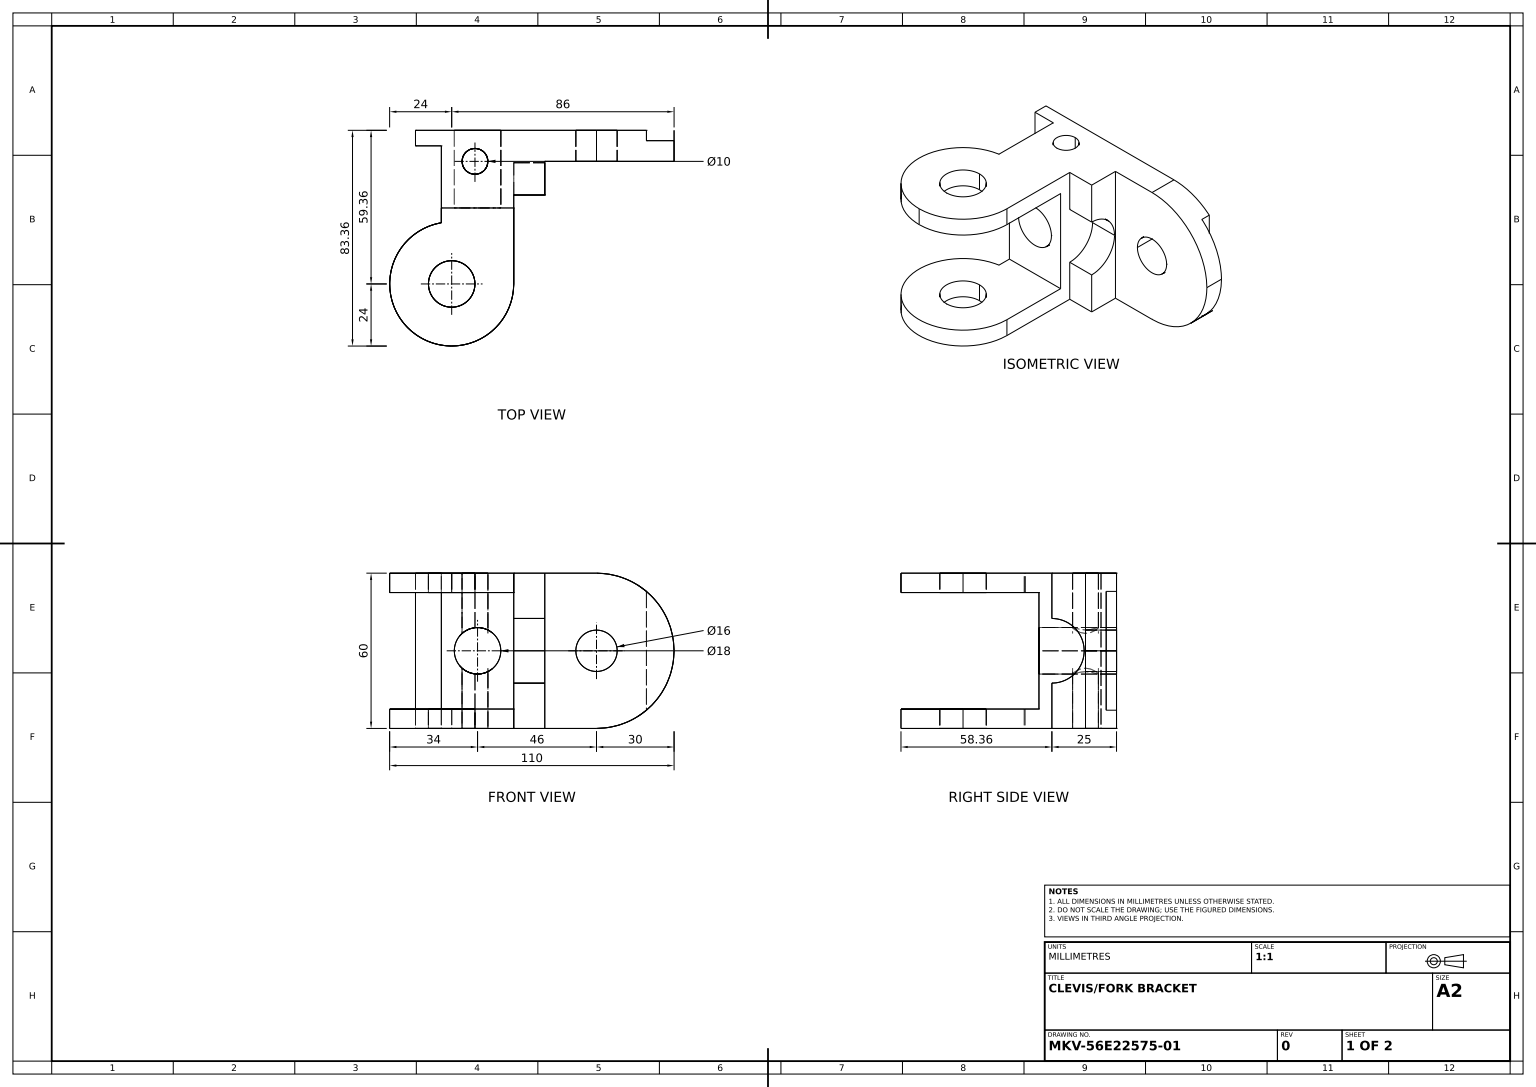
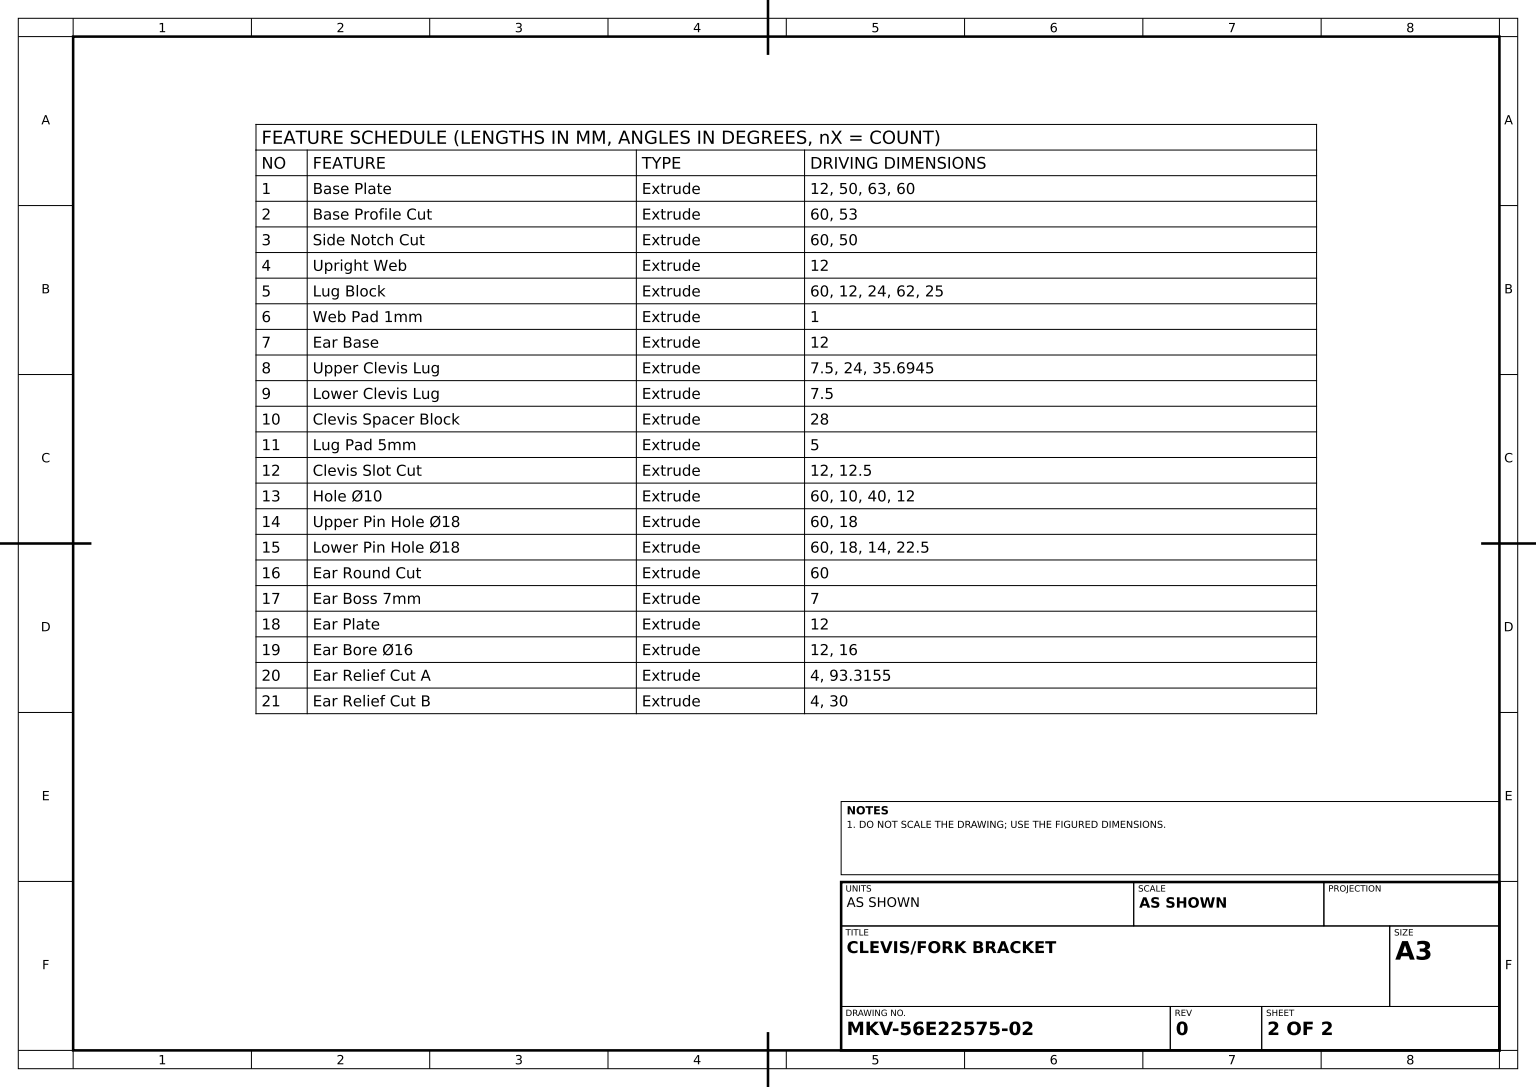
ISO-10303-21;
HEADER;
FILE_DESCRIPTION((''),'2;1');
FILE_NAME('','',(''),(''),'','','');
FILE_SCHEMA(('AUTOMOTIVE_DESIGN'));
ENDSEC;
DATA;
#1=APPLICATION_CONTEXT('');
#2=PRODUCT_CONTEXT('',#1,'mechanical');
#3=PRODUCT('','','',(#2));
#4=PRODUCT_DEFINITION_FORMATION('','',#3);
#5=PRODUCT_DEFINITION_CONTEXT('',#1,'design');
#6=PRODUCT_DEFINITION('','',#4,#5);
#7=PRODUCT_DEFINITION_SHAPE('','',#6);
#8=(LENGTH_UNIT()NAMED_UNIT(*)SI_UNIT(.MILLI.,.METRE.));
#9=(NAMED_UNIT(*)PLANE_ANGLE_UNIT()SI_UNIT($,.RADIAN.));
#10=(NAMED_UNIT(*)SI_UNIT($,.STERADIAN.)SOLID_ANGLE_UNIT());
#11=UNCERTAINTY_MEASURE_WITH_UNIT(LENGTH_MEASURE(1.E-05),#8,'distance_accuracy_value','');
#12=(GEOMETRIC_REPRESENTATION_CONTEXT(3)GLOBAL_UNCERTAINTY_ASSIGNED_CONTEXT((#11))GLOBAL_UNIT_ASSIGNED_CONTEXT((#8,#9,#10))REPRESENTATION_CONTEXT('',''));
#13=CARTESIAN_POINT('',(10.,52.5,35.694478));
#14=VERTEX_POINT('',#13);
#15=CARTESIAN_POINT('',(10.,60.,35.694478));
#16=VERTEX_POINT('',#15);
#17=DIRECTION('',(0.,1.,0.));
#18=VECTOR('',#17,1000.);
#19=LINE('',#13,#18);
#20=EDGE_CURVE('',#14,#16,#19,.T.);
#21=ORIENTED_EDGE('',*,*,#20,.T.);
#22=CARTESIAN_POINT('',(10.,60.,6.));
#23=VERTEX_POINT('',#22);
#24=CARTESIAN_POINT('',(10.,60.,0.));
#25=DIRECTION('',(0.,0.,1.));
#26=VECTOR('',#25,1000.);
#27=LINE('',#24,#26);
#28=EDGE_CURVE('',#23,#16,#27,.T.);
#29=ORIENTED_EDGE('',*,*,#28,.F.);
#30=CARTESIAN_POINT('',(10.,0.,6.));
#31=VERTEX_POINT('',#30);
#32=DIRECTION('',(0.,-1.,0.));
#33=VECTOR('',#32,1000.);
#34=LINE('',#22,#33);
#35=EDGE_CURVE('',#23,#31,#34,.T.);
#36=ORIENTED_EDGE('',*,*,#35,.T.);
#37=CARTESIAN_POINT('',(10.,0.,35.694478));
#38=VERTEX_POINT('',#37);
#39=CARTESIAN_POINT('',(10.,0.,0.));
#40=LINE('',#39,#26);
#41=EDGE_CURVE('',#31,#38,#40,.T.);
#42=ORIENTED_EDGE('',*,*,#41,.T.);
#43=CARTESIAN_POINT('',(10.,7.5,35.694478));
#44=VERTEX_POINT('',#43);
#45=LINE('',#43,#33);
#46=EDGE_CURVE('',#44,#38,#45,.T.);
#47=ORIENTED_EDGE('',*,*,#46,.F.);
#48=CARTESIAN_POINT('',(10.,7.5,30.));
#49=VERTEX_POINT('',#48);
#50=CARTESIAN_POINT('',(10.,7.5,0.));
#51=LINE('',#50,#26);
#52=EDGE_CURVE('',#49,#44,#51,.T.);
#53=ORIENTED_EDGE('',*,*,#52,.F.);
#54=CARTESIAN_POINT('',(10.,52.5,30.));
#55=VERTEX_POINT('',#54);
#56=LINE('',#48,#33);
#57=EDGE_CURVE('',#55,#49,#56,.T.);
#58=ORIENTED_EDGE('',*,*,#57,.F.);
#59=CARTESIAN_POINT('',(10.,52.5,12.));
#60=LINE('',#59,#26);
#61=EDGE_CURVE('',#55,#14,#60,.T.);
#62=ORIENTED_EDGE('',*,*,#61,.T.);
#63=EDGE_LOOP('',(#21,#29,#36,#42,#47,#53,#58,#62));
#64=FACE_OUTER_BOUND('',#63,.T.);
#65=DIRECTION('',(1.,0.,0.));
#66=DIRECTION('',(0.,0.,-1.));
#67=AXIS2_PLACEMENT_3D('',#24,#65,#66);
#68=PLANE('',#67);
#69=ADVANCED_FACE('',(#64),#68,.F.);
#70=CARTESIAN_POINT('',(38.,60.,25.));
#71=VERTEX_POINT('',#70);
#72=CARTESIAN_POINT('',(38.,42.5,25.));
#73=VERTEX_POINT('',#72);
#74=LINE('',#70,#33);
#75=EDGE_CURVE('',#71,#73,#74,.T.);
#76=ORIENTED_EDGE('',*,*,#75,.T.);
#77=CARTESIAN_POINT('',(50.,42.5,25.));
#78=VERTEX_POINT('',#77);
#79=VECTOR('',#65,1000.);
#80=LINE('',#72,#79);
#81=EDGE_CURVE('',#73,#78,#80,.T.);
#82=ORIENTED_EDGE('',*,*,#81,.T.);
#83=CARTESIAN_POINT('',(50.,60.,25.));
#84=VERTEX_POINT('',#83);
#85=LINE('',#83,#33);
#86=EDGE_CURVE('',#84,#78,#85,.T.);
#87=ORIENTED_EDGE('',*,*,#86,.F.);
#88=CARTESIAN_POINT('',(0.,60.,25.));
#89=DIRECTION('',(-1.,0.,0.));
#90=VECTOR('',#89,1000.);
#91=LINE('',#88,#90);
#92=EDGE_CURVE('',#84,#71,#91,.T.);
#93=ORIENTED_EDGE('',*,*,#92,.T.);
#94=EDGE_LOOP('',(#76,#82,#87,#93));
#95=FACE_OUTER_BOUND('',#94,.T.);
#96=AXIS2_PLACEMENT_3D('',#88,#25,#65);
#97=PLANE('',#96);
#98=ADVANCED_FACE('',(#95),#97,.T.);
#99=CARTESIAN_POINT('',(23.,21.055728,7.));
#100=VERTEX_POINT('',#99);
#101=CARTESIAN_POINT('',(23.,0.,7.));
#102=VERTEX_POINT('',#101);
#103=CARTESIAN_POINT('',(23.,60.,7.));
#104=LINE('',#103,#33);
#105=EDGE_CURVE('',#100,#102,#104,.T.);
#106=ORIENTED_EDGE('',*,*,#105,.T.);
#107=CARTESIAN_POINT('',(23.,0.,17.));
#108=VERTEX_POINT('',#107);
#109=CARTESIAN_POINT('',(23.,0.,12.));
#110=AXIS2_PLACEMENT_3D('',#109,#32,#66);
#111=CIRCLE('',#110,5.);
#112=EDGE_CURVE('',#102,#108,#111,.T.);
#113=ORIENTED_EDGE('',*,*,#112,.T.);
#114=CARTESIAN_POINT('',(23.,21.055728,17.));
#115=VERTEX_POINT('',#114);
#116=CARTESIAN_POINT('',(23.,60.,17.));
#117=LINE('',#116,#33);
#118=EDGE_CURVE('',#115,#108,#117,.T.);
#119=ORIENTED_EDGE('',*,*,#118,.F.);
#120=CARTESIAN_POINT('',(23.164559,21.03733,17.));
#121=CARTESIAN_POINT('',(23.331489,21.023356,16.991728));
#122=CARTESIAN_POINT('',(23.659912,21.004924,16.959007));
#123=CARTESIAN_POINT('',(23.822572,21.000307,16.934611));
#124=CARTESIAN_POINT('',(24.144827,20.999723,16.869946));
#125=CARTESIAN_POINT('',(24.304422,21.003758,16.829678));
#126=CARTESIAN_POINT('',(24.620491,21.02002,16.733003));
#127=CARTESIAN_POINT('',(24.777696,21.032359,16.676217));
#128=CARTESIAN_POINT('',(25.234199,21.079777,16.485219));
#129=CARTESIAN_POINT('',(25.521356,21.125209,16.330062));
#130=CARTESIAN_POINT('',(26.063223,21.235324,15.965266));
#131=CARTESIAN_POINT('',(26.316137,21.299898,15.755962));
#132=CARTESIAN_POINT('',(26.771191,21.433976,15.298808));
#133=CARTESIAN_POINT('',(26.977194,21.5045,15.047567));
#134=CARTESIAN_POINT('',(27.338414,21.639845,14.506771));
#135=CARTESIAN_POINT('',(27.490728,21.703413,14.222264));
#136=CARTESIAN_POINT('',(27.677746,21.785451,13.773404));
#137=CARTESIAN_POINT('',(27.733119,21.810578,13.620074));
#138=CARTESIAN_POINT('',(27.829366,21.855139,13.305481));
#139=CARTESIAN_POINT('',(27.870048,21.874484,13.144386));
#140=CARTESIAN_POINT('',(27.966967,21.921119,12.661194));
#141=CARTESIAN_POINT('',(27.999649,21.937568,12.335216));
#142=CARTESIAN_POINT('',(28.000171,21.937827,11.840298));
#143=CARTESIAN_POINT('',(27.992072,21.933793,11.673255));
#144=CARTESIAN_POINT('',(27.959417,21.917714,11.342939));
#145=CARTESIAN_POINT('',(27.93503,21.905755,11.180025));
#146=CARTESIAN_POINT('',(27.838546,21.859321,10.697691));
#147=CARTESIAN_POINT('',(27.742681,21.813959,10.383027));
#148=CARTESIAN_POINT('',(27.490749,21.703399,9.77721));
#149=CARTESIAN_POINT('',(27.337638,21.639562,9.492131));
#150=CARTESIAN_POINT('',(26.978581,21.505012,8.954446));
#151=CARTESIAN_POINT('',(26.770574,21.433771,8.700468));
#152=CARTESIAN_POINT('',(26.315151,21.299631,8.243152));
#153=CARTESIAN_POINT('',(26.066579,21.236114,8.037314));
#154=CARTESIAN_POINT('',(25.660178,21.153367,7.763238));
#155=CARTESIAN_POINT('',(25.51849,21.127826,7.677494));
#156=CARTESIAN_POINT('',(25.230085,21.083264,7.521879));
#157=CARTESIAN_POINT('',(25.082674,21.064075,7.451469));
#158=CARTESIAN_POINT('',(24.630812,21.017027,7.26216));
#159=CARTESIAN_POINT('',(24.316227,20.999606,7.164816));
#160=CARTESIAN_POINT('',(23.661717,21.000408,7.032748));
#161=CARTESIAN_POINT('',(23.330966,21.018725,7.));
#162=B_SPLINE_CURVE_WITH_KNOTS('',3,(#114,#120,#121,#122,#123,#124,#125,#126,#127,#128,#129,#130,#131,#132,#133,#134,#135,#136,#137,#138,#139,#140,#141,#142,#143,#144,#145,#146,#147,#148,#149,#150,#151,#152,#153,#154,#155,#156,#157,#158,#159,#160,#161,#99),.UNSPECIFIED.,.F.,.F.,(4,2,2,2,2,2,2,2,2,2,2,2,2,2,2,2,2,2,2,2,2,4),(0.016321692,0.01681327,0.017304849,0.017796427,0.018288006,0.019271163,0.02025432,0.021237477,0.022220634,0.022712213,0.023203791,0.024186948,0.024678527,0.025170106,0.026153263,0.02713642,0.028119577,0.029102734,0.029594313,0.030085891,0.031069048,0.032052205),.UNSPECIFIED.);
#163=EDGE_CURVE('',#115,#100,#162,.T.);
#164=ORIENTED_EDGE('',*,*,#163,.T.);
#165=EDGE_LOOP('',(#106,#113,#119,#164));
#166=FACE_OUTER_BOUND('',#165,.T.);
#167=CARTESIAN_POINT('',(23.,60.,12.));
#168=AXIS2_PLACEMENT_3D('',#167,#32,#66);
#169=CYLINDRICAL_SURFACE('',#168,5.);
#170=ADVANCED_FACE('',(#166),#169,.F.);
#171=CARTESIAN_POINT('',(15.,30.,0.));
#172=VERTEX_POINT('',#171);
#173=CARTESIAN_POINT('',(33.,30.,0.));
#174=VERTEX_POINT('',#173);
#175=CARTESIAN_POINT('',(24.,30.,0.));
#176=AXIS2_PLACEMENT_3D('',#175,#25,#65);
#177=CIRCLE('',#176,9.);
#178=EDGE_CURVE('',#172,#174,#177,.T.);
#179=ORIENTED_EDGE('',*,*,#178,.T.);
#180=EDGE_CURVE('',#174,#172,#177,.T.);
#181=ORIENTED_EDGE('',*,*,#180,.T.);
#182=EDGE_LOOP('',(#179,#181));
#183=FACE_BOUND('',#182,.T.);
#184=CARTESIAN_POINT('',(89.315471,52.954577,0.));
#185=VERTEX_POINT('',#184);
#186=CARTESIAN_POINT('',(70.,60.,0.));
#187=VERTEX_POINT('',#186);
#188=CARTESIAN_POINT('',(70.,30.,0.));
#189=AXIS2_PLACEMENT_3D('',#188,#25,#65);
#190=CIRCLE('',#189,30.);
#191=EDGE_CURVE('',#185,#187,#190,.T.);
#192=ORIENTED_EDGE('',*,*,#191,.F.);
#193=CARTESIAN_POINT('',(89.315471,7.045423,0.));
#194=VERTEX_POINT('',#193);
#195=CARTESIAN_POINT('',(89.315471,0.,0.));
#196=LINE('',#195,#33);
#197=EDGE_CURVE('',#185,#194,#196,.T.);
#198=ORIENTED_EDGE('',*,*,#197,.T.);
#199=CARTESIAN_POINT('',(70.,0.,0.));
#200=VERTEX_POINT('',#199);
#201=EDGE_CURVE('',#200,#194,#190,.T.);
#202=ORIENTED_EDGE('',*,*,#201,.F.);
#203=CARTESIAN_POINT('',(0.,0.,0.));
#204=VERTEX_POINT('',#203);
#205=CARTESIAN_POINT('',(50.,0.,0.));
#206=LINE('',#205,#79);
#207=EDGE_CURVE('',#204,#200,#206,.T.);
#208=ORIENTED_EDGE('',*,*,#207,.F.);
#209=CARTESIAN_POINT('',(0.,60.,0.));
#210=VERTEX_POINT('',#209);
#211=LINE('',#209,#33);
#212=EDGE_CURVE('',#210,#204,#211,.T.);
#213=ORIENTED_EDGE('',*,*,#212,.F.);
#214=CARTESIAN_POINT('',(50.,60.,0.));
#215=LINE('',#214,#90);
#216=EDGE_CURVE('',#187,#210,#215,.T.);
#217=ORIENTED_EDGE('',*,*,#216,.F.);
#218=EDGE_LOOP('',(#192,#198,#202,#208,#213,#217));
#219=FACE_OUTER_BOUND('',#218,.T.);
#220=CARTESIAN_POINT('',(62.,30.,0.));
#221=VERTEX_POINT('',#220);
#222=CARTESIAN_POINT('',(78.,30.,0.));
#223=VERTEX_POINT('',#222);
#224=CIRCLE('',#189,8.);
#225=EDGE_CURVE('',#221,#223,#224,.T.);
#226=ORIENTED_EDGE('',*,*,#225,.T.);
#227=EDGE_CURVE('',#223,#221,#224,.T.);
#228=ORIENTED_EDGE('',*,*,#227,.T.);
#229=EDGE_LOOP('',(#226,#228));
#230=FACE_BOUND('',#229,.T.);
#231=AXIS2_PLACEMENT_3D('',#203,#25,#65);
#232=PLANE('',#231);
#233=ADVANCED_FACE('',(#183,#219,#230),#232,.F.);
#234=CARTESIAN_POINT('',(50.,0.,12.));
#235=VERTEX_POINT('',#234);
#236=CARTESIAN_POINT('',(50.,0.,25.));
#237=VERTEX_POINT('',#236);
#238=LINE('',#205,#26);
#239=EDGE_CURVE('',#235,#237,#238,.T.);
#240=ORIENTED_EDGE('',*,*,#239,.T.);
#241=CARTESIAN_POINT('',(38.,0.,25.));
#242=VERTEX_POINT('',#241);
#243=CARTESIAN_POINT('',(0.,0.,25.));
#244=LINE('',#243,#90);
#245=EDGE_CURVE('',#237,#242,#244,.T.);
#246=ORIENTED_EDGE('',*,*,#245,.T.);
#247=CARTESIAN_POINT('',(38.,0.,59.358797));
#248=VERTEX_POINT('',#247);
#249=CARTESIAN_POINT('',(38.,0.,0.));
#250=VECTOR('',#66,1000.);
#251=LINE('',#249,#250);
#252=EDGE_CURVE('',#248,#242,#251,.T.);
#253=ORIENTED_EDGE('',*,*,#252,.F.);
#254=CARTESIAN_POINT('',(14.,0.,59.358797));
#255=AXIS2_PLACEMENT_3D('',#254,#32,#66);
#256=CIRCLE('',#255,24.);
#257=EDGE_CURVE('',#248,#38,#256,.T.);
#258=ORIENTED_EDGE('',*,*,#257,.T.);
#259=ORIENTED_EDGE('',*,*,#41,.F.);
#260=CARTESIAN_POINT('',(0.,0.,6.));
#261=VERTEX_POINT('',#260);
#262=LINE('',#260,#79);
#263=EDGE_CURVE('',#261,#31,#262,.T.);
#264=ORIENTED_EDGE('',*,*,#263,.F.);
#265=CARTESIAN_POINT('',(0.,0.,12.));
#266=LINE('',#265,#250);
#267=EDGE_CURVE('',#261,#204,#266,.T.);
#268=ORIENTED_EDGE('',*,*,#267,.T.);
#269=ORIENTED_EDGE('',*,*,#207,.T.);
#270=CARTESIAN_POINT('',(70.,0.,12.));
#271=VERTEX_POINT('',#270);
#272=LINE('',#199,#250);
#273=EDGE_CURVE('',#271,#200,#272,.T.);
#274=ORIENTED_EDGE('',*,*,#273,.F.);
#275=LINE('',#265,#79);
#276=EDGE_CURVE('',#235,#271,#275,.T.);
#277=ORIENTED_EDGE('',*,*,#276,.F.);
#278=EDGE_LOOP('',(#240,#246,#253,#258,#259,#264,#268,#269,#274,#277));
#279=FACE_OUTER_BOUND('',#278,.T.);
#280=EDGE_CURVE('',#108,#102,#111,.T.);
#281=ORIENTED_EDGE('',*,*,#280,.F.);
#282=ORIENTED_EDGE('',*,*,#112,.F.);
#283=EDGE_LOOP('',(#281,#282));
#284=FACE_BOUND('',#283,.T.);
#285=CARTESIAN_POINT('',(14.,0.,50.358797));
#286=VERTEX_POINT('',#285);
#287=CARTESIAN_POINT('',(14.,0.,68.358797));
#288=VERTEX_POINT('',#287);
#289=CIRCLE('',#255,9.);
#290=EDGE_CURVE('',#286,#288,#289,.T.);
#291=ORIENTED_EDGE('',*,*,#290,.F.);
#292=EDGE_CURVE('',#288,#286,#289,.T.);
#293=ORIENTED_EDGE('',*,*,#292,.F.);
#294=EDGE_LOOP('',(#291,#293));
#295=FACE_BOUND('',#294,.T.);
#296=AXIS2_PLACEMENT_3D('',#234,#17,#25);
#297=PLANE('',#296);
#298=ADVANCED_FACE('',(#279,#284,#295),#297,.F.);
#299=CARTESIAN_POINT('',(50.,17.5,25.));
#300=VERTEX_POINT('',#299);
#301=CARTESIAN_POINT('',(50.,30.,12.5));
#302=VERTEX_POINT('',#301);
#303=CARTESIAN_POINT('',(50.,30.,25.));
#304=AXIS2_PLACEMENT_3D('',#303,#65,#66);
#305=CIRCLE('',#304,12.5);
#306=EDGE_CURVE('',#300,#302,#305,.T.);
#307=ORIENTED_EDGE('',*,*,#306,.T.);
#308=CARTESIAN_POINT('',(38.,30.,12.5));
#309=VERTEX_POINT('',#308);
#310=LINE('',#308,#79);
#311=EDGE_CURVE('',#309,#302,#310,.T.);
#312=ORIENTED_EDGE('',*,*,#311,.F.);
#313=CARTESIAN_POINT('',(38.,17.5,25.));
#314=VERTEX_POINT('',#313);
#315=CARTESIAN_POINT('',(38.,30.,25.));
#316=AXIS2_PLACEMENT_3D('',#315,#65,#66);
#317=CIRCLE('',#316,12.5);
#318=EDGE_CURVE('',#314,#309,#317,.T.);
#319=ORIENTED_EDGE('',*,*,#318,.F.);
#320=LINE('',#313,#79);
#321=EDGE_CURVE('',#314,#300,#320,.T.);
#322=ORIENTED_EDGE('',*,*,#321,.T.);
#323=EDGE_LOOP('',(#307,#312,#319,#322));
#324=FACE_OUTER_BOUND('',#323,.T.);
#325=CYLINDRICAL_SURFACE('',#316,12.5);
#326=ADVANCED_FACE('',(#324),#325,.F.);
#327=CARTESIAN_POINT('',(33.,30.,30.));
#328=VERTEX_POINT('',#327);
#329=CARTESIAN_POINT('',(15.,30.,30.));
#330=VERTEX_POINT('',#329);
#331=CARTESIAN_POINT('',(24.,30.,30.));
#332=AXIS2_PLACEMENT_3D('',#331,#25,#65);
#333=CIRCLE('',#332,9.);
#334=EDGE_CURVE('',#328,#330,#333,.T.);
#335=ORIENTED_EDGE('',*,*,#334,.F.);
#336=EDGE_CURVE('',#330,#328,#333,.T.);
#337=ORIENTED_EDGE('',*,*,#336,.F.);
#338=EDGE_LOOP('',(#335,#337));
#339=FACE_BOUND('',#338,.T.);
#340=ORIENTED_EDGE('',*,*,#57,.T.);
#341=CARTESIAN_POINT('',(38.,7.5,30.));
#342=VERTEX_POINT('',#341);
#343=LINE('',#341,#79);
#344=EDGE_CURVE('',#49,#342,#343,.T.);
#345=ORIENTED_EDGE('',*,*,#344,.T.);
#346=CARTESIAN_POINT('',(38.,52.5,30.));
#347=VERTEX_POINT('',#346);
#348=LINE('',#346,#18);
#349=EDGE_CURVE('',#342,#347,#348,.T.);
#350=ORIENTED_EDGE('',*,*,#349,.T.);
#351=LINE('',#54,#90);
#352=EDGE_CURVE('',#347,#55,#351,.T.);
#353=ORIENTED_EDGE('',*,*,#352,.T.);
#354=EDGE_LOOP('',(#340,#345,#350,#353));
#355=FACE_OUTER_BOUND('',#354,.T.);
#356=CARTESIAN_POINT('',(0.,0.,30.));
#357=AXIS2_PLACEMENT_3D('',#356,#66,#89);
#358=PLANE('',#357);
#359=ADVANCED_FACE('',(#339,#355),#358,.F.);
#360=CARTESIAN_POINT('',(14.,7.5,68.358797));
#361=VERTEX_POINT('',#360);
#362=CARTESIAN_POINT('',(14.,60.,68.358797));
#363=LINE('',#362,#33);
#364=EDGE_CURVE('',#361,#288,#363,.T.);
#365=ORIENTED_EDGE('',*,*,#364,.F.);
#366=CARTESIAN_POINT('',(14.,7.5,50.358797));
#367=VERTEX_POINT('',#366);
#368=CARTESIAN_POINT('',(14.,7.5,59.358797));
#369=AXIS2_PLACEMENT_3D('',#368,#32,#66);
#370=CIRCLE('',#369,9.);
#371=EDGE_CURVE('',#367,#361,#370,.T.);
#372=ORIENTED_EDGE('',*,*,#371,.F.);
#373=CARTESIAN_POINT('',(14.,60.,50.358797));
#374=LINE('',#373,#33);
#375=EDGE_CURVE('',#367,#286,#374,.T.);
#376=ORIENTED_EDGE('',*,*,#375,.T.);
#377=ORIENTED_EDGE('',*,*,#290,.T.);
#378=EDGE_LOOP('',(#365,#372,#376,#377));
#379=FACE_OUTER_BOUND('',#378,.T.);
#380=CARTESIAN_POINT('',(14.,60.,59.358797));
#381=AXIS2_PLACEMENT_3D('',#380,#32,#66);
#382=CYLINDRICAL_SURFACE('',#381,9.);
#383=ADVANCED_FACE('',(#379),#382,.F.);
#384=ORIENTED_EDGE('',*,*,#292,.T.);
#385=ORIENTED_EDGE('',*,*,#375,.F.);
#386=EDGE_CURVE('',#361,#367,#370,.T.);
#387=ORIENTED_EDGE('',*,*,#386,.F.);
#388=ORIENTED_EDGE('',*,*,#364,.T.);
#389=EDGE_LOOP('',(#384,#385,#387,#388));
#390=FACE_OUTER_BOUND('',#389,.T.);
#391=ADVANCED_FACE('',(#390),#382,.F.);
#392=CARTESIAN_POINT('',(23.,38.944272,7.));
#393=VERTEX_POINT('',#392);
#394=CARTESIAN_POINT('',(23.,38.944272,17.));
#395=VERTEX_POINT('',#394);
#396=CARTESIAN_POINT('',(23.331952,38.981385,7.));
#397=CARTESIAN_POINT('',(23.659425,38.999354,7.032736));
#398=CARTESIAN_POINT('',(24.305537,39.000612,7.162219));
#399=CARTESIAN_POINT('',(24.627248,38.983287,7.260796));
#400=CARTESIAN_POINT('',(25.233528,38.920274,7.514541));
#401=CARTESIAN_POINT('',(25.521043,38.874889,7.669624));
#402=CARTESIAN_POINT('',(26.065706,38.764137,8.036509));
#403=CARTESIAN_POINT('',(26.31626,38.700075,8.244117));
#404=CARTESIAN_POINT('',(26.771747,38.56585,8.701795));
#405=CARTESIAN_POINT('',(26.979409,38.4947,8.955488));
#406=CARTESIAN_POINT('',(27.338692,38.36002,9.493908));
#407=CARTESIAN_POINT('',(27.491066,38.296452,9.77823));
#408=CARTESIAN_POINT('',(27.741204,38.186699,10.379221));
#409=CARTESIAN_POINT('',(27.838619,38.140644,10.698122));
#410=CARTESIAN_POINT('',(27.967042,38.07884,11.33999));
#411=CARTESIAN_POINT('',(27.999905,38.062305,11.666379));
#412=CARTESIAN_POINT('',(28.000047,38.062234,12.164667));
#413=CARTESIAN_POINT('',(27.991702,38.06639,12.331934));
#414=CARTESIAN_POINT('',(27.958921,38.082529,12.660587));
#415=CARTESIAN_POINT('',(27.934511,38.094498,12.823088));
#416=CARTESIAN_POINT('',(27.837738,38.141062,13.305298));
#417=CARTESIAN_POINT('',(27.740526,38.187021,13.623006));
#418=CARTESIAN_POINT('',(27.489024,38.297323,14.226072));
#419=CARTESIAN_POINT('',(27.335846,38.361177,14.511128));
#420=CARTESIAN_POINT('',(26.974855,38.496316,15.050549));
#421=CARTESIAN_POINT('',(26.767231,38.567308,15.303315));
#422=CARTESIAN_POINT('',(26.311856,38.701244,15.759725));
#423=CARTESIAN_POINT('',(26.062229,38.764979,15.966236));
#424=CARTESIAN_POINT('',(25.516042,38.875768,16.333336));
#425=CARTESIAN_POINT('',(25.228729,38.920883,16.487716));
#426=CARTESIAN_POINT('',(24.776332,38.967736,16.676682));
#427=CARTESIAN_POINT('',(24.621937,38.979882,16.732513));
#428=CARTESIAN_POINT('',(24.305612,38.996204,16.829362));
#429=CARTESIAN_POINT('',(24.142793,39.000334,16.87047));
#430=CARTESIAN_POINT('',(23.65538,38.999268,16.967926));
#431=CARTESIAN_POINT('',(23.328562,38.981006,17.));
#432=B_SPLINE_CURVE_WITH_KNOTS('',3,(#392,#396,#397,#398,#399,#400,#401,#402,#403,#404,#405,#406,#407,#408,#409,#410,#411,#412,#413,#414,#415,#416,#417,#418,#419,#420,#421,#422,#423,#424,#425,#426,#427,#428,#429,#430,#431,#394),.UNSPECIFIED.,.F.,.F.,(4,2,2,2,2,2,2,2,2,2,2,2,2,2,2,2,2,2,4),(0.,0.000987077,0.001974153,0.00296123,0.003948307,0.004935384,0.00592246,0.006909537,0.007896614,0.008390152,0.008883691,0.009870767,0.010857844,0.011844921,0.012831998,0.013819074,0.014312613,0.014806151,0.015793228),.UNSPECIFIED.);
#433=EDGE_CURVE('',#393,#395,#432,.T.);
#434=ORIENTED_EDGE('',*,*,#433,.F.);
#435=CARTESIAN_POINT('',(22.83034,38.925303,17.));
#436=CARTESIAN_POINT('',(22.659097,38.901188,16.991235));
#437=CARTESIAN_POINT('',(22.322403,38.843915,16.956763));
#438=CARTESIAN_POINT('',(22.156886,38.810836,16.931206));
#439=CARTESIAN_POINT('',(21.668349,38.699139,16.830865));
#440=CARTESIAN_POINT('',(21.350501,38.607059,16.731364));
#441=CARTESIAN_POINT('',(20.749084,38.398384,16.476609));
#442=CARTESIAN_POINT('',(20.467453,38.282894,16.322981));
#443=CARTESIAN_POINT('',(19.938125,38.036566,15.965713));
#444=CARTESIAN_POINT('',(19.691194,37.90574,15.76177));
#445=CARTESIAN_POINT('',(19.245487,37.645988,15.317038));
#446=CARTESIAN_POINT('',(19.044184,37.515846,15.074755));
#447=CARTESIAN_POINT('',(18.684189,37.265687,14.544872));
#448=CARTESIAN_POINT('',(18.529357,37.148331,14.262518));
#449=CARTESIAN_POINT('',(18.337892,36.996226,13.814154));
#450=CARTESIAN_POINT('',(18.280756,36.949424,13.660267));
#451=CARTESIAN_POINT('',(18.180707,36.865863,13.34245));
#452=CARTESIAN_POINT('',(18.137989,36.829266,13.178636));
#453=CARTESIAN_POINT('',(18.035599,36.740481,12.684146));
#454=CARTESIAN_POINT('',(17.999961,36.708169,12.344143));
#455=CARTESIAN_POINT('',(18.00004,36.708239,11.65471));
#456=CARTESIAN_POINT('',(18.03532,36.740238,11.317332));
#457=CARTESIAN_POINT('',(18.138007,36.829282,10.82121));
#458=CARTESIAN_POINT('',(18.180835,36.865971,10.657131));
#459=CARTESIAN_POINT('',(18.280694,36.949372,10.339941));
#460=CARTESIAN_POINT('',(18.33789,36.996229,10.185778));
#461=CARTESIAN_POINT('',(18.53037,37.149126,9.735252));
#462=CARTESIAN_POINT('',(18.687657,37.26819,9.4495));
#463=CARTESIAN_POINT('',(19.045957,37.516983,8.923167));
#464=CARTESIAN_POINT('',(19.247782,37.647531,8.680002));
#465=CARTESIAN_POINT('',(19.699573,37.910413,8.230556));
#466=CARTESIAN_POINT('',(19.943633,38.03928,8.030213));
#467=CARTESIAN_POINT('',(20.338202,38.222668,7.764439));
#468=CARTESIAN_POINT('',(20.474514,38.282165,7.681688));
#469=CARTESIAN_POINT('',(20.757411,38.396959,7.528234));
#470=CARTESIAN_POINT('',(20.904909,38.452565,7.457163));
#471=CARTESIAN_POINT('',(21.35714,38.609128,7.266281));
#472=CARTESIAN_POINT('',(21.669516,38.699385,7.168932));
#473=CARTESIAN_POINT('',(22.155499,38.810529,7.06906));
#474=CARTESIAN_POINT('',(22.320412,38.843531,7.04352));
#475=CARTESIAN_POINT('',(22.65649,38.900789,7.008954));
#476=CARTESIAN_POINT('',(22.82859,38.925108,7.));
#477=B_SPLINE_CURVE_WITH_KNOTS('',3,(#394,#435,#436,#437,#438,#439,#440,#441,#442,#443,#444,#445,#446,#447,#448,#449,#450,#451,#452,#453,#454,#455,#456,#457,#458,#459,#460,#461,#462,#463,#464,#465,#466,#467,#468,#469,#470,#471,#472,#473,#474,#475,#476,#392),.UNSPECIFIED.,.F.,.F.,(4,2,2,2,2,2,2,2,2,2,2,2,2,2,2,2,2,2,2,2,2,4),(0.015793228,0.016302925,0.016812623,0.017832017,0.018851412,0.019870807,0.020890202,0.021909596,0.022419294,0.022928991,0.023948386,0.02496778,0.025477478,0.025987175,0.02700657,0.028025965,0.029045359,0.029555057,0.030064754,0.031084149,0.031593846,0.032103544),.UNSPECIFIED.);
#478=EDGE_CURVE('',#395,#393,#477,.T.);
#479=ORIENTED_EDGE('',*,*,#478,.F.);
#480=EDGE_LOOP('',(#434,#479));
#481=FACE_BOUND('',#480,.T.);
#482=ORIENTED_EDGE('',*,*,#334,.T.);
#483=CARTESIAN_POINT('',(15.,30.,-30.));
#484=LINE('',#483,#26);
#485=EDGE_CURVE('',#172,#330,#484,.T.);
#486=ORIENTED_EDGE('',*,*,#485,.F.);
#487=ORIENTED_EDGE('',*,*,#180,.F.);
#488=CARTESIAN_POINT('',(33.,30.,-30.));
#489=LINE('',#488,#26);
#490=EDGE_CURVE('',#174,#328,#489,.T.);
#491=ORIENTED_EDGE('',*,*,#490,.T.);
#492=EDGE_LOOP('',(#482,#486,#487,#491));
#493=FACE_OUTER_BOUND('',#492,.T.);
#494=CARTESIAN_POINT('',(24.,30.,-30.));
#495=AXIS2_PLACEMENT_3D('',#494,#25,#65);
#496=CYLINDRICAL_SURFACE('',#495,9.);
#497=ADVANCED_FACE('',(#481,#493),#496,.F.);
#498=CARTESIAN_POINT('',(14.,52.5,50.358797));
#499=VERTEX_POINT('',#498);
#500=CARTESIAN_POINT('',(14.,52.5,68.358797));
#501=VERTEX_POINT('',#500);
#502=CARTESIAN_POINT('',(14.,52.5,59.358797));
#503=AXIS2_PLACEMENT_3D('',#502,#17,#25);
#504=CIRCLE('',#503,9.);
#505=EDGE_CURVE('',#499,#501,#504,.T.);
#506=ORIENTED_EDGE('',*,*,#505,.T.);
#507=EDGE_CURVE('',#501,#499,#504,.T.);
#508=ORIENTED_EDGE('',*,*,#507,.T.);
#509=EDGE_LOOP('',(#506,#508));
#510=FACE_BOUND('',#509,.T.);
#511=CARTESIAN_POINT('',(14.,52.5,83.358797));
#512=VERTEX_POINT('',#511);
#513=CARTESIAN_POINT('',(38.,52.5,59.358797));
#514=VERTEX_POINT('',#513);
#515=CIRCLE('',#503,24.);
#516=EDGE_CURVE('',#512,#514,#515,.T.);
#517=ORIENTED_EDGE('',*,*,#516,.F.);
#518=EDGE_CURVE('',#14,#512,#515,.T.);
#519=ORIENTED_EDGE('',*,*,#518,.F.);
#520=ORIENTED_EDGE('',*,*,#61,.F.);
#521=ORIENTED_EDGE('',*,*,#352,.F.);
#522=CARTESIAN_POINT('',(38.,52.5,12.));
#523=LINE('',#522,#250);
#524=EDGE_CURVE('',#514,#347,#523,.T.);
#525=ORIENTED_EDGE('',*,*,#524,.F.);
#526=EDGE_LOOP('',(#517,#519,#520,#521,#525));
#527=FACE_OUTER_BOUND('',#526,.T.);
#528=PLANE('',#503);
#529=ADVANCED_FACE('',(#510,#527),#528,.F.);
#530=ORIENTED_EDGE('',*,*,#433,.T.);
#531=VERTEX_POINT('',#116);
#532=EDGE_CURVE('',#531,#395,#117,.T.);
#533=ORIENTED_EDGE('',*,*,#532,.F.);
#534=VERTEX_POINT('',#103);
#535=CIRCLE('',#168,5.);
#536=EDGE_CURVE('',#534,#531,#535,.T.);
#537=ORIENTED_EDGE('',*,*,#536,.F.);
#538=EDGE_CURVE('',#534,#393,#104,.T.);
#539=ORIENTED_EDGE('',*,*,#538,.T.);
#540=EDGE_LOOP('',(#530,#533,#537,#539));
#541=FACE_OUTER_BOUND('',#540,.T.);
#542=ADVANCED_FACE('',(#541),#169,.F.);
#543=CARTESIAN_POINT('',(89.315471,52.954577,4.));
#544=VERTEX_POINT('',#543);
#545=CARTESIAN_POINT('',(100.,30.,4.));
#546=VERTEX_POINT('',#545);
#547=CARTESIAN_POINT('',(70.,30.,4.));
#548=AXIS2_PLACEMENT_3D('',#547,#66,#89);
#549=CIRCLE('',#548,30.);
#550=EDGE_CURVE('',#544,#546,#549,.T.);
#551=ORIENTED_EDGE('',*,*,#550,.T.);
#552=CARTESIAN_POINT('',(89.315471,7.045423,4.));
#553=VERTEX_POINT('',#552);
#554=EDGE_CURVE('',#546,#553,#549,.T.);
#555=ORIENTED_EDGE('',*,*,#554,.T.);
#556=CARTESIAN_POINT('',(89.315471,0.,4.));
#557=LINE('',#556,#33);
#558=EDGE_CURVE('',#544,#553,#557,.T.);
#559=ORIENTED_EDGE('',*,*,#558,.F.);
#560=EDGE_LOOP('',(#551,#555,#559));
#561=FACE_OUTER_BOUND('',#560,.T.);
#562=PLANE('',#548);
#563=ADVANCED_FACE('',(#561),#562,.T.);
#564=CARTESIAN_POINT('',(100.,30.,12.));
#565=VERTEX_POINT('',#564);
#566=CARTESIAN_POINT('',(100.,30.,0.));
#567=LINE('',#566,#26);
#568=EDGE_CURVE('',#546,#565,#567,.T.);
#569=ORIENTED_EDGE('',*,*,#568,.F.);
#570=ORIENTED_EDGE('',*,*,#550,.F.);
#571=LINE('',#543,#250);
#572=EDGE_CURVE('',#544,#185,#571,.T.);
#573=ORIENTED_EDGE('',*,*,#572,.T.);
#574=ORIENTED_EDGE('',*,*,#191,.T.);
#575=CARTESIAN_POINT('',(70.,60.,12.));
#576=VERTEX_POINT('',#575);
#577=LINE('',#575,#26);
#578=EDGE_CURVE('',#187,#576,#577,.T.);
#579=ORIENTED_EDGE('',*,*,#578,.T.);
#580=CARTESIAN_POINT('',(70.,30.,12.));
#581=AXIS2_PLACEMENT_3D('',#580,#25,#65);
#582=CIRCLE('',#581,30.);
#583=EDGE_CURVE('',#565,#576,#582,.T.);
#584=ORIENTED_EDGE('',*,*,#583,.F.);
#585=EDGE_LOOP('',(#569,#570,#573,#574,#579,#584));
#586=FACE_OUTER_BOUND('',#585,.T.);
#587=CYLINDRICAL_SURFACE('',#189,30.);
#588=ADVANCED_FACE('',(#586),#587,.T.);
#589=ORIENTED_EDGE('',*,*,#225,.F.);
#590=CARTESIAN_POINT('',(62.,30.,12.));
#591=VERTEX_POINT('',#590);
#592=LINE('',#220,#26);
#593=EDGE_CURVE('',#221,#591,#592,.T.);
#594=ORIENTED_EDGE('',*,*,#593,.T.);
#595=CARTESIAN_POINT('',(78.,30.,12.));
#596=VERTEX_POINT('',#595);
#597=CIRCLE('',#581,8.);
#598=EDGE_CURVE('',#591,#596,#597,.T.);
#599=ORIENTED_EDGE('',*,*,#598,.T.);
#600=LINE('',#222,#26);
#601=EDGE_CURVE('',#223,#596,#600,.T.);
#602=ORIENTED_EDGE('',*,*,#601,.F.);
#603=EDGE_LOOP('',(#589,#594,#599,#602));
#604=FACE_OUTER_BOUND('',#603,.T.);
#605=CYLINDRICAL_SURFACE('',#189,8.);
#606=ADVANCED_FACE('',(#604),#605,.F.);
#607=EDGE_CURVE('',#302,#78,#305,.T.);
#608=ORIENTED_EDGE('',*,*,#607,.T.);
#609=ORIENTED_EDGE('',*,*,#81,.F.);
#610=EDGE_CURVE('',#309,#73,#317,.T.);
#611=ORIENTED_EDGE('',*,*,#610,.F.);
#612=ORIENTED_EDGE('',*,*,#311,.T.);
#613=EDGE_LOOP('',(#608,#609,#611,#612));
#614=FACE_OUTER_BOUND('',#613,.T.);
#615=ADVANCED_FACE('',(#614),#325,.F.);
#616=CARTESIAN_POINT('',(0.,60.,6.));
#617=VERTEX_POINT('',#616);
#618=LINE('',#616,#79);
#619=EDGE_CURVE('',#617,#23,#618,.T.);
#620=ORIENTED_EDGE('',*,*,#619,.F.);
#621=LINE('',#616,#33);
#622=EDGE_CURVE('',#617,#261,#621,.T.);
#623=ORIENTED_EDGE('',*,*,#622,.T.);
#624=ORIENTED_EDGE('',*,*,#263,.T.);
#625=ORIENTED_EDGE('',*,*,#35,.F.);
#626=EDGE_LOOP('',(#620,#623,#624,#625));
#627=FACE_OUTER_BOUND('',#626,.T.);
#628=AXIS2_PLACEMENT_3D('',#616,#66,#89);
#629=PLANE('',#628);
#630=ADVANCED_FACE('',(#627),#629,.F.);
#631=ORIENTED_EDGE('',*,*,#252,.T.);
#632=EDGE_CURVE('',#314,#242,#74,.T.);
#633=ORIENTED_EDGE('',*,*,#632,.F.);
#634=ORIENTED_EDGE('',*,*,#318,.T.);
#635=ORIENTED_EDGE('',*,*,#610,.T.);
#636=ORIENTED_EDGE('',*,*,#75,.F.);
#637=CARTESIAN_POINT('',(38.,60.,59.358797));
#638=VERTEX_POINT('',#637);
#639=CARTESIAN_POINT('',(38.,60.,12.));
#640=LINE('',#639,#250);
#641=EDGE_CURVE('',#638,#71,#640,.T.);
#642=ORIENTED_EDGE('',*,*,#641,.F.);
#643=LINE('',#513,#18);
#644=EDGE_CURVE('',#514,#638,#643,.T.);
#645=ORIENTED_EDGE('',*,*,#644,.F.);
#646=ORIENTED_EDGE('',*,*,#524,.T.);
#647=ORIENTED_EDGE('',*,*,#349,.F.);
#648=CARTESIAN_POINT('',(38.,7.5,59.358797));
#649=VERTEX_POINT('',#648);
#650=CARTESIAN_POINT('',(38.,7.5,0.));
#651=LINE('',#650,#250);
#652=EDGE_CURVE('',#649,#342,#651,.T.);
#653=ORIENTED_EDGE('',*,*,#652,.F.);
#654=LINE('',#648,#33);
#655=EDGE_CURVE('',#649,#248,#654,.T.);
#656=ORIENTED_EDGE('',*,*,#655,.T.);
#657=EDGE_LOOP('',(#631,#633,#634,#635,#636,#642,#645,#646,#647,#653,#656));
#658=FACE_OUTER_BOUND('',#657,.T.);
#659=AXIS2_PLACEMENT_3D('',#650,#89,#25);
#660=PLANE('',#659);
#661=ADVANCED_FACE('',(#658),#660,.F.);
#662=VERTEX_POINT('',#362);
#663=VERTEX_POINT('',#373);
#664=CIRCLE('',#381,9.);
#665=EDGE_CURVE('',#662,#663,#664,.T.);
#666=ORIENTED_EDGE('',*,*,#665,.F.);
#667=EDGE_CURVE('',#662,#501,#363,.T.);
#668=ORIENTED_EDGE('',*,*,#667,.T.);
#669=ORIENTED_EDGE('',*,*,#505,.F.);
#670=EDGE_CURVE('',#663,#499,#374,.T.);
#671=ORIENTED_EDGE('',*,*,#670,.F.);
#672=EDGE_LOOP('',(#666,#668,#669,#671));
#673=FACE_OUTER_BOUND('',#672,.T.);
#674=ADVANCED_FACE('',(#673),#382,.F.);
#675=ORIENTED_EDGE('',*,*,#306,.F.);
#676=EDGE_CURVE('',#300,#237,#85,.T.);
#677=ORIENTED_EDGE('',*,*,#676,.T.);
#678=ORIENTED_EDGE('',*,*,#239,.F.);
#679=CARTESIAN_POINT('',(50.,60.,12.));
#680=VERTEX_POINT('',#679);
#681=LINE('',#679,#33);
#682=EDGE_CURVE('',#680,#235,#681,.T.);
#683=ORIENTED_EDGE('',*,*,#682,.F.);
#684=LINE('',#214,#26);
#685=EDGE_CURVE('',#680,#84,#684,.T.);
#686=ORIENTED_EDGE('',*,*,#685,.T.);
#687=ORIENTED_EDGE('',*,*,#86,.T.);
#688=ORIENTED_EDGE('',*,*,#607,.F.);
#689=EDGE_LOOP('',(#675,#677,#678,#683,#686,#687,#688));
#690=FACE_OUTER_BOUND('',#689,.T.);
#691=AXIS2_PLACEMENT_3D('',#214,#65,#66);
#692=PLANE('',#691);
#693=ADVANCED_FACE('',(#690),#692,.T.);
#694=CARTESIAN_POINT('',(14.,60.,83.358797));
#695=VERTEX_POINT('',#694);
#696=AXIS2_PLACEMENT_3D('',#380,#17,#25);
#697=CIRCLE('',#696,24.);
#698=EDGE_CURVE('',#695,#638,#697,.T.);
#699=ORIENTED_EDGE('',*,*,#698,.F.);
#700=LINE('',#511,#18);
#701=EDGE_CURVE('',#512,#695,#700,.T.);
#702=ORIENTED_EDGE('',*,*,#701,.F.);
#703=ORIENTED_EDGE('',*,*,#516,.T.);
#704=ORIENTED_EDGE('',*,*,#644,.T.);
#705=EDGE_LOOP('',(#699,#702,#703,#704));
#706=FACE_OUTER_BOUND('',#705,.T.);
#707=CYLINDRICAL_SURFACE('',#503,24.);
#708=ADVANCED_FACE('',(#706),#707,.T.);
#709=ORIENTED_EDGE('',*,*,#163,.F.);
#710=CARTESIAN_POINT('',(22.656595,21.094122,7.));
#711=CARTESIAN_POINT('',(22.322611,21.151395,7.034971));
#712=CARTESIAN_POINT('',(21.67167,21.299981,7.168239));
#713=CARTESIAN_POINT('',(21.351659,21.392619,7.268301));
#714=CARTESIAN_POINT('',(20.751944,21.600544,7.522026));
#715=CARTESIAN_POINT('',(20.470001,21.71598,7.67544));
#716=CARTESIAN_POINT('',(19.938589,21.963159,8.033834));
#717=CARTESIAN_POINT('',(19.692843,22.093355,8.236767));
#718=CARTESIAN_POINT('',(19.246724,22.353236,8.681547));
#719=CARTESIAN_POINT('',(19.04351,22.484609,8.926159));
#720=CARTESIAN_POINT('',(18.684085,22.7344,9.455361));
#721=CARTESIAN_POINT('',(18.530655,22.850687,9.735154));
#722=CARTESIAN_POINT('',(18.339779,23.00225,10.181076));
#723=CARTESIAN_POINT('',(18.28276,23.048928,10.334129));
#724=CARTESIAN_POINT('',(18.18278,23.132381,10.650233));
#725=CARTESIAN_POINT('',(18.139602,23.169347,10.814594));
#726=CARTESIAN_POINT('',(18.036038,23.259116,11.311742));
#727=CARTESIAN_POINT('',(18.00031,23.291519,11.649911));
#728=CARTESIAN_POINT('',(17.999694,23.29207,12.34118));
#729=CARTESIAN_POINT('',(18.035188,23.259882,12.681631));
#730=CARTESIAN_POINT('',(18.137713,23.170971,13.177565));
#731=CARTESIAN_POINT('',(18.180551,23.134268,13.341915));
#732=CARTESIAN_POINT('',(18.280703,23.050619,13.660137));
#733=CARTESIAN_POINT('',(18.337924,23.003746,13.814265));
#734=CARTESIAN_POINT('',(18.529778,22.851339,14.263437));
#735=CARTESIAN_POINT('',(18.685227,22.73354,14.546696));
#736=CARTESIAN_POINT('',(19.046086,22.482886,15.077254));
#737=CARTESIAN_POINT('',(19.248183,22.352285,15.320236));
#738=CARTESIAN_POINT('',(19.696619,22.091257,15.766666));
#739=CARTESIAN_POINT('',(19.945231,21.959874,15.971107));
#740=CARTESIAN_POINT('',(20.473418,21.714591,16.326394));
#741=CARTESIAN_POINT('',(20.754324,21.599628,16.479157));
#742=CARTESIAN_POINT('',(21.353899,21.391934,16.732469));
#743=CARTESIAN_POINT('',(21.675019,21.299096,16.832661));
#744=CARTESIAN_POINT('',(22.325501,21.150857,16.965404));
#745=CARTESIAN_POINT('',(22.658513,21.093908,17.));
#746=B_SPLINE_CURVE_WITH_KNOTS('',3,(#99,#710,#711,#712,#713,#714,#715,#716,#717,#718,#719,#720,#721,#722,#723,#724,#725,#726,#727,#728,#729,#730,#731,#732,#733,#734,#735,#736,#737,#738,#739,#740,#741,#742,#743,#744,#745,#114),.UNSPECIFIED.,.F.,.F.,(4,2,2,2,2,2,2,2,2,2,2,2,2,2,2,2,2,2,4),(0.,0.001020106,0.002040211,0.003060317,0.004080423,0.005100529,0.006120634,0.006630687,0.00714074,0.008160846,0.009180952,0.009691004,0.010201057,0.011221163,0.012241269,0.013261374,0.01428148,0.015301586,0.016321692),.UNSPECIFIED.);
#747=EDGE_CURVE('',#100,#115,#746,.T.);
#748=ORIENTED_EDGE('',*,*,#747,.F.);
#749=EDGE_LOOP('',(#709,#748));
#750=FACE_BOUND('',#749,.T.);
#751=ORIENTED_EDGE('',*,*,#485,.T.);
#752=ORIENTED_EDGE('',*,*,#336,.T.);
#753=ORIENTED_EDGE('',*,*,#490,.F.);
#754=ORIENTED_EDGE('',*,*,#178,.F.);
#755=EDGE_LOOP('',(#751,#752,#753,#754));
#756=FACE_OUTER_BOUND('',#755,.T.);
#757=ADVANCED_FACE('',(#750,#756),#496,.F.);
#758=EDGE_CURVE('',#16,#695,#697,.T.);
#759=ORIENTED_EDGE('',*,*,#758,.F.);
#760=ORIENTED_EDGE('',*,*,#20,.F.);
#761=ORIENTED_EDGE('',*,*,#518,.T.);
#762=ORIENTED_EDGE('',*,*,#701,.T.);
#763=EDGE_LOOP('',(#759,#760,#761,#762));
#764=FACE_OUTER_BOUND('',#763,.T.);
#765=ADVANCED_FACE('',(#764),#707,.T.);
#766=ORIENTED_EDGE('',*,*,#52,.T.);
#767=CIRCLE('',#369,24.);
#768=EDGE_CURVE('',#649,#44,#767,.T.);
#769=ORIENTED_EDGE('',*,*,#768,.F.);
#770=ORIENTED_EDGE('',*,*,#652,.T.);
#771=ORIENTED_EDGE('',*,*,#344,.F.);
#772=EDGE_LOOP('',(#766,#769,#770,#771));
#773=FACE_OUTER_BOUND('',#772,.T.);
#774=ORIENTED_EDGE('',*,*,#371,.T.);
#775=ORIENTED_EDGE('',*,*,#386,.T.);
#776=EDGE_LOOP('',(#774,#775));
#777=FACE_BOUND('',#776,.T.);
#778=CARTESIAN_POINT('',(0.,7.5,0.));
#779=AXIS2_PLACEMENT_3D('',#778,#32,#66);
#780=PLANE('',#779);
#781=ADVANCED_FACE('',(#773,#777),#780,.F.);
#782=ORIENTED_EDGE('',*,*,#572,.F.);
#783=ORIENTED_EDGE('',*,*,#558,.T.);
#784=LINE('',#552,#250);
#785=EDGE_CURVE('',#553,#194,#784,.T.);
#786=ORIENTED_EDGE('',*,*,#785,.T.);
#787=ORIENTED_EDGE('',*,*,#197,.F.);
#788=EDGE_LOOP('',(#782,#783,#786,#787));
#789=FACE_OUTER_BOUND('',#788,.T.);
#790=AXIS2_PLACEMENT_3D('',#556,#65,#66);
#791=PLANE('',#790);
#792=ADVANCED_FACE('',(#789),#791,.T.);
#793=ORIENTED_EDGE('',*,*,#583,.T.);
#794=CARTESIAN_POINT('',(63.,60.,12.));
#795=LINE('',#794,#90);
#796=EDGE_CURVE('',#576,#680,#795,.T.);
#797=ORIENTED_EDGE('',*,*,#796,.T.);
#798=ORIENTED_EDGE('',*,*,#682,.T.);
#799=ORIENTED_EDGE('',*,*,#276,.T.);
#800=EDGE_CURVE('',#271,#565,#582,.T.);
#801=ORIENTED_EDGE('',*,*,#800,.T.);
#802=EDGE_LOOP('',(#793,#797,#798,#799,#801));
#803=FACE_OUTER_BOUND('',#802,.T.);
#804=ORIENTED_EDGE('',*,*,#598,.F.);
#805=EDGE_CURVE('',#596,#591,#597,.T.);
#806=ORIENTED_EDGE('',*,*,#805,.F.);
#807=EDGE_LOOP('',(#804,#806));
#808=FACE_BOUND('',#807,.T.);
#809=AXIS2_PLACEMENT_3D('',#265,#25,#65);
#810=PLANE('',#809);
#811=ADVANCED_FACE('',(#803,#808),#810,.T.);
#812=ORIENTED_EDGE('',*,*,#280,.T.);
#813=ORIENTED_EDGE('',*,*,#105,.F.);
#814=ORIENTED_EDGE('',*,*,#747,.T.);
#815=ORIENTED_EDGE('',*,*,#118,.T.);
#816=EDGE_LOOP('',(#812,#813,#814,#815));
#817=FACE_OUTER_BOUND('',#816,.T.);
#818=ADVANCED_FACE('',(#817),#169,.F.);
#819=ORIENTED_EDGE('',*,*,#46,.T.);
#820=ORIENTED_EDGE('',*,*,#257,.F.);
#821=ORIENTED_EDGE('',*,*,#655,.F.);
#822=ORIENTED_EDGE('',*,*,#768,.T.);
#823=EDGE_LOOP('',(#819,#820,#821,#822));
#824=FACE_OUTER_BOUND('',#823,.T.);
#825=CYLINDRICAL_SURFACE('',#369,24.);
#826=ADVANCED_FACE('',(#824),#825,.T.);
#827=EDGE_CURVE('',#663,#662,#664,.T.);
#828=ORIENTED_EDGE('',*,*,#827,.F.);
#829=ORIENTED_EDGE('',*,*,#670,.T.);
#830=ORIENTED_EDGE('',*,*,#507,.F.);
#831=ORIENTED_EDGE('',*,*,#667,.F.);
#832=EDGE_LOOP('',(#828,#829,#830,#831));
#833=FACE_OUTER_BOUND('',#832,.T.);
#834=ADVANCED_FACE('',(#833),#382,.F.);
#835=ORIENTED_EDGE('',*,*,#227,.F.);
#836=ORIENTED_EDGE('',*,*,#601,.T.);
#837=ORIENTED_EDGE('',*,*,#805,.T.);
#838=ORIENTED_EDGE('',*,*,#593,.F.);
#839=EDGE_LOOP('',(#835,#836,#837,#838));
#840=FACE_OUTER_BOUND('',#839,.T.);
#841=ADVANCED_FACE('',(#840),#605,.F.);
#842=ORIENTED_EDGE('',*,*,#538,.F.);
#843=EDGE_CURVE('',#531,#534,#535,.T.);
#844=ORIENTED_EDGE('',*,*,#843,.F.);
#845=ORIENTED_EDGE('',*,*,#532,.T.);
#846=ORIENTED_EDGE('',*,*,#478,.T.);
#847=EDGE_LOOP('',(#842,#844,#845,#846));
#848=FACE_OUTER_BOUND('',#847,.T.);
#849=ADVANCED_FACE('',(#848),#169,.F.);
#850=ORIENTED_EDGE('',*,*,#568,.T.);
#851=ORIENTED_EDGE('',*,*,#800,.F.);
#852=ORIENTED_EDGE('',*,*,#273,.T.);
#853=ORIENTED_EDGE('',*,*,#201,.T.);
#854=ORIENTED_EDGE('',*,*,#785,.F.);
#855=ORIENTED_EDGE('',*,*,#554,.F.);
#856=EDGE_LOOP('',(#850,#851,#852,#853,#854,#855));
#857=FACE_OUTER_BOUND('',#856,.T.);
#858=ADVANCED_FACE('',(#857),#587,.T.);
#859=ORIENTED_EDGE('',*,*,#578,.F.);
#860=ORIENTED_EDGE('',*,*,#216,.T.);
#861=CARTESIAN_POINT('',(0.,60.,12.));
#862=LINE('',#861,#250);
#863=EDGE_CURVE('',#617,#210,#862,.T.);
#864=ORIENTED_EDGE('',*,*,#863,.F.);
#865=ORIENTED_EDGE('',*,*,#619,.T.);
#866=ORIENTED_EDGE('',*,*,#28,.T.);
#867=ORIENTED_EDGE('',*,*,#758,.T.);
#868=ORIENTED_EDGE('',*,*,#698,.T.);
#869=ORIENTED_EDGE('',*,*,#641,.T.);
#870=ORIENTED_EDGE('',*,*,#92,.F.);
#871=ORIENTED_EDGE('',*,*,#685,.F.);
#872=ORIENTED_EDGE('',*,*,#796,.F.);
#873=EDGE_LOOP('',(#859,#860,#864,#865,#866,#867,#868,#869,#870,#871,#872));
#874=FACE_OUTER_BOUND('',#873,.T.);
#875=ORIENTED_EDGE('',*,*,#843,.T.);
#876=ORIENTED_EDGE('',*,*,#536,.T.);
#877=EDGE_LOOP('',(#875,#876));
#878=FACE_BOUND('',#877,.T.);
#879=ORIENTED_EDGE('',*,*,#827,.T.);
#880=ORIENTED_EDGE('',*,*,#665,.T.);
#881=EDGE_LOOP('',(#879,#880));
#882=FACE_BOUND('',#881,.T.);
#883=AXIS2_PLACEMENT_3D('',#679,#32,#66);
#884=PLANE('',#883);
#885=ADVANCED_FACE('',(#874,#878,#882),#884,.F.);
#886=ORIENTED_EDGE('',*,*,#212,.T.);
#887=ORIENTED_EDGE('',*,*,#267,.F.);
#888=ORIENTED_EDGE('',*,*,#622,.F.);
#889=ORIENTED_EDGE('',*,*,#863,.T.);
#890=EDGE_LOOP('',(#886,#887,#888,#889));
#891=FACE_OUTER_BOUND('',#890,.T.);
#892=AXIS2_PLACEMENT_3D('',#861,#65,#66);
#893=PLANE('',#892);
#894=ADVANCED_FACE('',(#891),#893,.F.);
#895=ORIENTED_EDGE('',*,*,#632,.T.);
#896=ORIENTED_EDGE('',*,*,#245,.F.);
#897=ORIENTED_EDGE('',*,*,#676,.F.);
#898=ORIENTED_EDGE('',*,*,#321,.F.);
#899=EDGE_LOOP('',(#895,#896,#897,#898));
#900=FACE_OUTER_BOUND('',#899,.T.);
#901=ADVANCED_FACE('',(#900),#97,.T.);
#902=CLOSED_SHELL('',(#69,#98,#170,#233,#298,#326,#359,#383,#391,#497,#529,#542,#563,#588,#606,#615,#630,#661,#674,#693,#708,#757,#765,#781,#792,#811,#818,#826,#834,#841,#849,#858,#885,#894,#901));
#903=MANIFOLD_SOLID_BREP('',#902);
#904=ADVANCED_BREP_SHAPE_REPRESENTATION('',(#903),#12);
#905=SHAPE_DEFINITION_REPRESENTATION(#7,#904);
ENDSEC;
END-ISO-10303-21;
